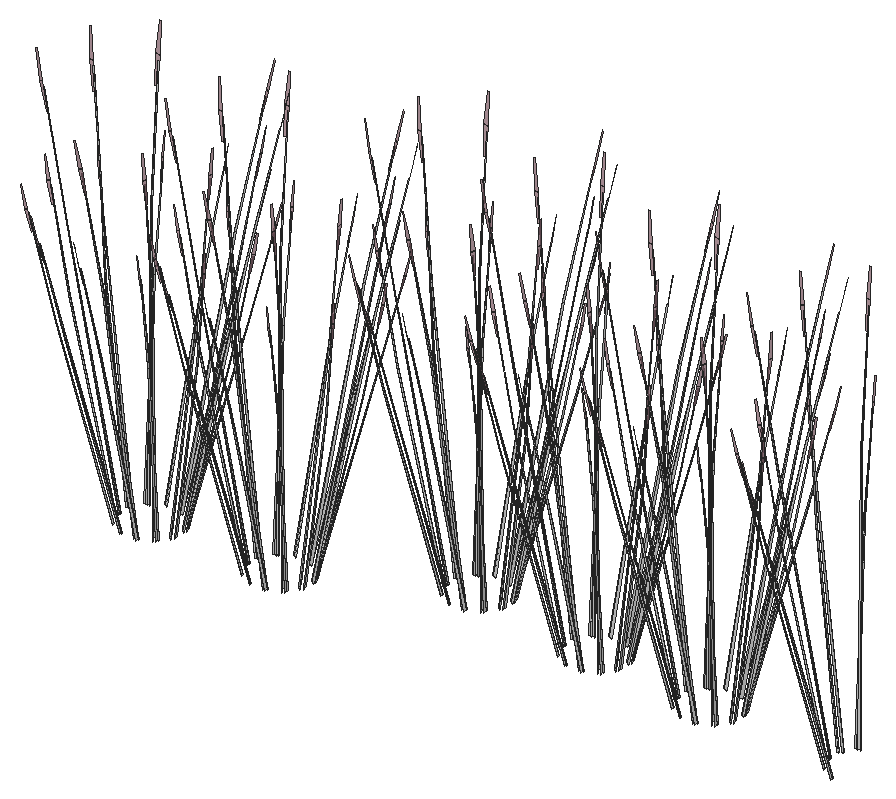
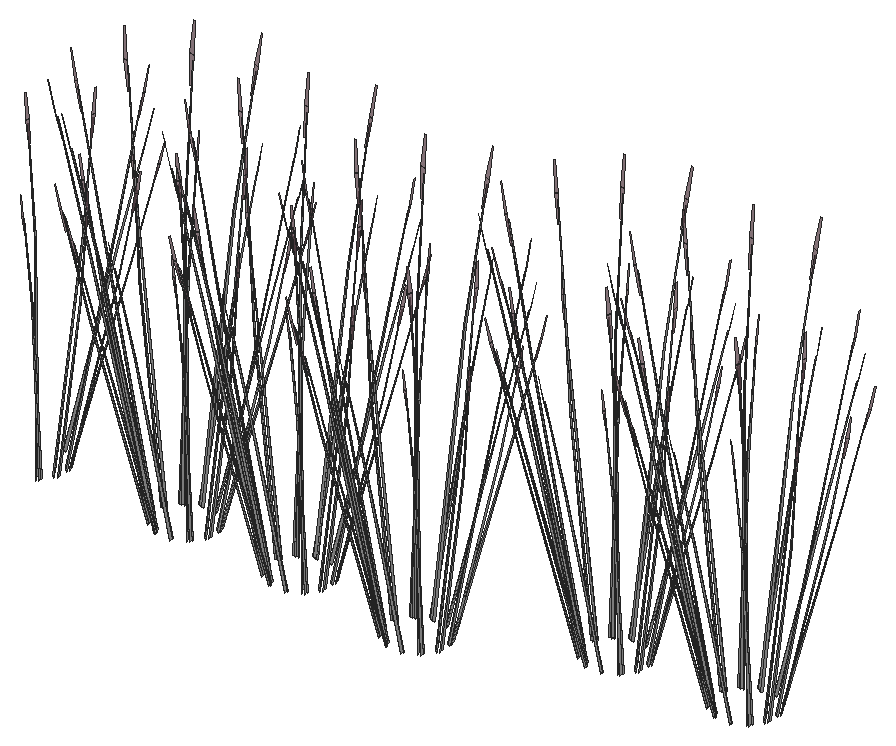
# SketchUp Ruby script. Lengths in inches.
U = 1.inch
M = Sketchup.active_model
def pt(a) = Geom::Point3d.new(a.map { |v| v * U })
def face(e, loops, mat)
  f = e.add_face(loops[0].map { |a| pt(a) })
  loops[1..].each { |l| e.add_face(l.map { |a| pt(a) }).erase! }
  f.material = f.back_material = mat if mat
  f
end
# faces: each face lists its corners as indices into pts; further lists are holes
def faces(e, pts, list, mat = nil) = list.each { |f| face(e, (f[0].is_a?(Array) ? f : [f]).map { |l| l.map { |i| pts[i] } }, mat) }
# xy, xz, yz: faces in a plane at the given z, y or x. An outline is a flat list of corners, or four numbers for a rectangle; further outlines are holes
def ring(l) = l.size == 4 ? [[l[0], l[1]], [l[2], l[1]], [l[2], l[3]], [l[0], l[3]]] : l.each_slice(2).to_a
def flat(e, list, mat, &to3) = list.each { |f| face(e, (f[0].is_a?(Array) ? f : [f]).map { |l| ring(l).map { |u, v| to3.(u, v) } }, mat) }
def xy(e, z, list, mat = nil) = flat(e, list, mat) { |x, y| [x, y, z] }
def xz(e, y, list, mat = nil) = flat(e, list, mat) { |x, z| [x, y, z] }
def yz(e, x, list, mat = nil) = flat(e, list, mat) { |y, z| [x, y, z] }
def lines(e, pts, list) = list.each { |a, b| e.add_line(pt(pts[a]), pt(pts[b])) }
# prism: a flat outline (further loops are holes) pulled along v
def prism(e, loops, v, mat = nil)
  f = face(e, loops, mat); d = Geom::Vector3d.new(v.map { |x| x * U })
  f.pushpull(f.normal.samedirection?(d) ? d.length : -d.length)
end
def box(e, o, s, mat = nil) = prism(e, [[o, [o[0] + s[0], o[1], o[2]], [o[0] + s[0], o[1] + s[1], o[2]], [o[0], o[1] + s[1], o[2]]]], [0, 0, s[2]], mat)
def at(x, y, z, deg = 0) = Geom::Transformation.translation(pt([x, y, z])) * Geom::Transformation.rotation(ORIGIN, Z_AXIS, deg.degrees)
def axes(o, x, y, z) = Geom::Transformation.new([*x, 0, *y, 0, *z, 0, *pt(o).to_a, 1])
def part(name) = M.definitions.add(name)
# library, detail: a bought-in or finely detailed component or shape, given as its bounding box
def library(name, o, s) = part(name).tap { |d| box(d.entities, o, s) }
def detail(e, o, s) = box(e.add_group.entities, o, s)
def put(e, d, t, mat = nil) = e.add_instance(d, t).tap { |i| i.material = mat if mat }
def group(e, t, mat = nil) = e.add_group.tap { |g| g.transformation = t; g.material = mat if mat }.entities
root = M.entities
M.materials.add("LightPink_Translucent").color = [144, 107, 117]
M.materials["LightPink_Translucent"].alpha = 0.75
M.materials.add("[_0053_Ivory_]").color = [200, 200, 200]
c1 = part("blade")
p = [[2.15,0.21,22],[0,0.17,0],[0.09,0.45,0],[2.18,0.31,22],[2.29,0.31,22],[0.38,0.45,0],
  [2.48,0.24,33],[2.49,0.24,33],[2.48,0.22,33]]
faces(c1.entities,p,[[0,1,2,3],[4,5,2,3],[6,3,4,7],[8,0,3,6]])
c2 = part("seeds")
p = [[0.3,-0.1,1.38],[-0.01,-0.03,1.59],[-0.01,-0.03,0.03],[0.14,-0.07,-0.07],[0.29,-0.03,3],[0.15,0.01,3.11]]
faces(c2.entities,p,[[0,1,2,3],[1,0,4,5]],"LightPink_Translucent")
c3 = part("blade with seeds")
put(c3.entities,c1,at(0,0,0))
put(c3.entities,c2,axes([2.4,0.25,30.99],[1.5799,-0.05474,1.17369],[-0.12525,1.92788,0.29478],[-0.07173,-0.02425,1.56792]))
put(root,c3,axes([417.64,97.95,131.39],[0.17159,-0.57338,0.48003],[0.56413,0.19607,0.3958],[-0.22185,0.03446,0.9933]),"[_0053_Ivory_]")
put(root,c3,axes([417.59,97.8,131.38],[-0.22307,-0.42878,0.0643],[0.40677,-0.20987,0.50621],[-0.17931,0.04141,0.77189]),"[_0053_Ivory_]")
put(root,c3,axes([417.77,99.38,131.39],[-0.15063,-0.57876,0.48003],[0.59087,-0.10045,0.3958],[-0.17414,0.13612,0.9933]),"[_0053_Ivory_]")
put(root,c3,axes([417.66,99.27,131.38],[-0.41695,-0.26447,0.0643],[0.24275,-0.37662,0.50621],[-0.13368,0.12176,0.77189]),"[_0053_Ivory_]")
put(root,c3,axes([418.31,96.5,131.38],[0.03058,-0.47819,0.0643],[0.4618,0.01311,0.50621],[-0.1769,-0.05004,0.77189]),"[_0053_Ivory_]")
put(root,c3,axes([418.64,100.55,131.39],[-0.43249,-0.42907,0.48003],[0.45929,-0.37004,0.3958],[-0.07978,0.2013,0.9933]),"[_0053_Ivory_]")
put(root,c3,axes([418.48,100.51,131.38],[-0.49911,-0.0293,0.0643],[0.01368,-0.44245,0.50621],[-0.05223,0.16948,0.77189]),"[_0053_Ivory_]")
put(root,c3,axes([419.6,95.71,131.38],[0.27604,-0.39948,0.0643],[0.39309,0.23258,0.50621],[-0.12709,-0.12808,0.77189]),"[_0053_Ivory_]")
put(root,c3,axes([419.84,101.2,131.38],[-0.44753,0.21372,0.0643],[-0.21905,-0.38973,0.50621],[0.04322,0.1718,0.77189]),"[_0053_Ivory_]")
put(root,c3,axes([421.14,95.65,131.38],[0.44753,-0.21372,0.0643],[0.21905,0.38973,0.50621],[-0.04322,-0.1718,0.77189]),"[_0053_Ivory_]")
put(root,c3,axes([420.98,95.7,131.39],[0.59846,0.1644,0.48003],[-0.20464,0.54049,0.3958],[-0.03596,-0.21255,0.9933]),"[_0053_Ivory_]")
put(root,c3,axes([421.48,101.02,131.39],[-0.60408,0.14432,0.48003],[-0.10484,-0.56611,0.3958],[0.14207,0.16684,0.9933]),"[_0053_Ivory_]")
put(root,c3,axes([421.37,101.14,131.38],[-0.27604,0.39948,0.0643],[-0.39309,-0.23258,0.50621],[0.12709,0.12808,0.77189]),"[_0053_Ivory_]")
put(root,c3,axes([422.49,96.34,131.38],[0.49911,0.0293,0.0643],[-0.01368,0.44245,0.50621],[0.05223,-0.16948,0.77189]),"[_0053_Ivory_]")
put(root,c3,axes([422.34,96.3,131.39],[0.43249,0.42907,0.48003],[-0.45929,0.37004,0.3958],[0.07978,-0.2013,0.9933]),"[_0053_Ivory_]")
put(root,c3,axes([422.67,100.35,131.38],[-0.03058,0.47819,0.0643],[-0.4618,-0.01311,0.50621],[0.1769,0.05004,0.77189]),"[_0053_Ivory_]")
put(root,c3,axes([422.71,100.2,131.39],[-0.44783,0.41436,0.48003],[-0.38623,-0.44004,0.3958],[0.21011,0.07643,0.9933]),"[_0053_Ivory_]")
put(root,c3,axes([429.85,97.95,131.39],[0.17159,-0.57338,0.48003],[0.56413,0.19607,0.3958],[-0.22185,0.03446,0.9933]),"[_0053_Ivory_]")
put(root,c3,axes([423.32,97.58,131.38],[0.41695,0.26447,0.0643],[-0.24275,0.37662,0.50621],[0.13368,-0.12176,0.77189]),"[_0053_Ivory_]")
put(root,c3,axes([429.81,97.8,131.38],[-0.22307,-0.42878,0.0643],[0.40677,-0.20987,0.50621],[-0.17931,0.04141,0.77189]),"[_0053_Ivory_]")
put(root,c3,axes([423.2,97.47,131.39],[0.15063,0.57876,0.48003],[-0.59087,0.10045,0.3958],[0.17414,-0.13612,0.9933]),"[_0053_Ivory_]")
put(root,c3,axes([429.99,99.38,131.39],[-0.15063,-0.57876,0.48003],[0.59087,-0.10045,0.3958],[-0.17414,0.13612,0.9933]),"[_0053_Ivory_]")
put(root,c3,axes([423.38,99.05,131.38],[0.22307,0.42878,0.0643],[-0.40677,0.20987,0.50621],[0.17931,-0.04141,0.77189]),"[_0053_Ivory_]")
put(root,c3,axes([429.87,99.27,131.38],[-0.41695,-0.26447,0.0643],[0.24275,-0.37662,0.50621],[-0.13368,0.12176,0.77189]),"[_0053_Ivory_]")
put(root,c3,axes([423.33,98.9,131.39],[-0.17159,0.57338,0.48003],[-0.56413,-0.19607,0.3958],[0.22185,-0.03446,0.9933]),"[_0053_Ivory_]")
put(root,c3,axes([430.52,96.5,131.38],[0.03058,-0.47819,0.0643],[0.4618,0.01311,0.50621],[-0.1769,-0.05004,0.77189]),"[_0053_Ivory_]")
put(root,c3,axes([430.85,100.55,131.39],[-0.43249,-0.42907,0.48003],[0.45929,-0.37004,0.3958],[-0.07978,0.2013,0.9933]),"[_0053_Ivory_]")
put(root,c3,axes([430.69,100.51,131.38],[-0.49911,-0.0293,0.0643],[0.01368,-0.44245,0.50621],[-0.05223,0.16948,0.77189]),"[_0053_Ivory_]")
put(root,c3,axes([431.82,95.71,131.38],[0.27604,-0.39948,0.0643],[0.39309,0.23258,0.50621],[-0.12709,-0.12808,0.77189]),"[_0053_Ivory_]")
put(root,c3,axes([432.05,101.2,131.38],[-0.44753,0.21372,0.0643],[-0.21905,-0.38973,0.50621],[0.04322,0.1718,0.77189]),"[_0053_Ivory_]")
put(root,c3,axes([433.35,95.65,131.38],[0.44753,-0.21372,0.0643],[0.21905,0.38973,0.50621],[-0.04322,-0.1718,0.77189]),"[_0053_Ivory_]")
put(root,c3,axes([433.19,95.7,131.39],[0.59846,0.1644,0.48003],[-0.20464,0.54049,0.3958],[-0.03596,-0.21255,0.9933]),"[_0053_Ivory_]")
put(root,c3,axes([433.7,101.02,131.39],[-0.60408,0.14432,0.48003],[-0.10484,-0.56611,0.3958],[0.14207,0.16684,0.9933]),"[_0053_Ivory_]")
put(root,c3,axes([433.58,101.14,131.38],[-0.27604,0.39948,0.0643],[-0.39309,-0.23258,0.50621],[0.12709,0.12808,0.77189]),"[_0053_Ivory_]")
put(root,c3,axes([434.71,96.34,131.38],[0.49911,0.0293,0.0643],[-0.01368,0.44245,0.50621],[0.05223,-0.16948,0.77189]),"[_0053_Ivory_]")
put(root,c3,axes([434.55,96.3,131.39],[0.43249,0.42907,0.48003],[-0.45929,0.37004,0.3958],[0.07978,-0.2013,0.9933]),"[_0053_Ivory_]")
put(root,c3,axes([434.88,100.35,131.38],[-0.03058,0.47819,0.0643],[-0.4618,-0.01311,0.50621],[0.1769,0.05004,0.77189]),"[_0053_Ivory_]")
put(root,c3,axes([434.92,100.2,131.39],[-0.44783,0.41436,0.48003],[-0.38623,-0.44004,0.3958],[0.21011,0.07643,0.9933]),"[_0053_Ivory_]")
put(root,c3,axes([435.53,97.58,131.38],[0.41695,0.26447,0.0643],[-0.24275,0.37662,0.50621],[0.13368,-0.12176,0.77189]),"[_0053_Ivory_]")
put(root,c3,axes([435.41,97.47,131.39],[0.15063,0.57876,0.48003],[-0.59087,0.10045,0.3958],[0.17414,-0.13612,0.9933]),"[_0053_Ivory_]")
put(root,c3,axes([435.59,99.05,131.38],[0.22307,0.42878,0.0643],[-0.40677,0.20987,0.50621],[0.17931,-0.04141,0.77189]),"[_0053_Ivory_]")
put(root,c3,axes([435.55,98.9,131.39],[-0.17159,0.57338,0.48003],[-0.56413,-0.19607,0.3958],[0.22185,-0.03446,0.9933]),"[_0053_Ivory_]")
put(root,c3,axes([443.25,104.76,131.39],[0.17159,-0.57338,0.48003],[0.56413,0.19607,0.3958],[-0.22185,0.03446,0.9933]),"[_0053_Ivory_]")
put(root,c3,axes([443.21,104.61,131.38],[-0.22307,-0.42878,0.0643],[0.40677,-0.20987,0.50621],[-0.17931,0.04141,0.77189]),"[_0053_Ivory_]")
put(root,c3,axes([443.39,106.19,131.39],[-0.15063,-0.57876,0.48003],[0.59087,-0.10045,0.3958],[-0.17414,0.13612,0.9933]),"[_0053_Ivory_]")
put(root,c3,axes([443.27,106.08,131.38],[-0.41695,-0.26447,0.0643],[0.24275,-0.37662,0.50621],[-0.13368,0.12176,0.77189]),"[_0053_Ivory_]")
put(root,c3,axes([443.92,103.31,131.38],[0.03058,-0.47819,0.0643],[0.4618,0.01311,0.50621],[-0.1769,-0.05004,0.77189]),"[_0053_Ivory_]")
put(root,c3,axes([444.25,107.36,131.39],[-0.43249,-0.42907,0.48003],[0.45929,-0.37004,0.3958],[-0.07978,0.2013,0.9933]),"[_0053_Ivory_]")
put(root,c3,axes([444.09,107.32,131.38],[-0.49911,-0.0293,0.0643],[0.01368,-0.44245,0.50621],[-0.05223,0.16948,0.77189]),"[_0053_Ivory_]")
put(root,c3,axes([445.22,102.52,131.38],[0.27604,-0.39948,0.0643],[0.39309,0.23258,0.50621],[-0.12709,-0.12808,0.77189]),"[_0053_Ivory_]")
put(root,c3,axes([445.45,108.01,131.38],[-0.44753,0.21372,0.0643],[-0.21905,-0.38973,0.50621],[0.04322,0.1718,0.77189]),"[_0053_Ivory_]")
put(root,c3,axes([446.75,102.46,131.38],[0.44753,-0.21372,0.0643],[0.21905,0.38973,0.50621],[-0.04322,-0.1718,0.77189]),"[_0053_Ivory_]")
put(root,c3,axes([446.59,102.5,131.39],[0.59846,0.1644,0.48003],[-0.20464,0.54049,0.3958],[-0.03596,-0.21255,0.9933]),"[_0053_Ivory_]")
put(root,c3,axes([447.1,107.83,131.39],[-0.60408,0.14432,0.48003],[-0.10484,-0.56611,0.3958],[0.14207,0.16684,0.9933]),"[_0053_Ivory_]")
put(root,c3,axes([446.99,107.95,131.38],[-0.27604,0.39948,0.0643],[-0.39309,-0.23258,0.50621],[0.12709,0.12808,0.77189]),"[_0053_Ivory_]")
put(root,c3,axes([448.11,103.15,131.38],[0.49911,0.0293,0.0643],[-0.01368,0.44245,0.50621],[0.05223,-0.16948,0.77189]),"[_0053_Ivory_]")
put(root,c3,axes([447.95,103.11,131.39],[0.43249,0.42907,0.48003],[-0.45929,0.37004,0.3958],[0.07978,-0.2013,0.9933]),"[_0053_Ivory_]")
put(root,c3,axes([448.28,107.16,131.38],[-0.03058,0.47819,0.0643],[-0.4618,-0.01311,0.50621],[0.1769,0.05004,0.77189]),"[_0053_Ivory_]")
put(root,c3,axes([448.32,107.01,131.39],[-0.44783,0.41436,0.48003],[-0.38623,-0.44004,0.3958],[0.21011,0.07643,0.9933]),"[_0053_Ivory_]")
put(root,c3,axes([448.93,104.39,131.38],[0.41695,0.26447,0.0643],[-0.24275,0.37662,0.50621],[0.13368,-0.12176,0.77189]),"[_0053_Ivory_]")
put(root,c3,axes([448.82,104.28,131.39],[0.15063,0.57876,0.48003],[-0.59087,0.10045,0.3958],[0.17414,-0.13612,0.9933]),"[_0053_Ivory_]")
put(root,c3,axes([455.74,102.94,131.39],[0.17159,-0.57338,0.48003],[0.56413,0.19607,0.3958],[-0.22185,0.03446,0.9933]),"[_0053_Ivory_]")
put(root,c3,axes([455.69,102.79,131.38],[-0.22307,-0.42878,0.0643],[0.40677,-0.20987,0.50621],[-0.17931,0.04141,0.77189]),"[_0053_Ivory_]")
put(root,c3,axes([448.99,105.86,131.38],[0.22307,0.42878,0.0643],[-0.40677,0.20987,0.50621],[0.17931,-0.04141,0.77189]),"[_0053_Ivory_]")
put(root,c3,axes([448.95,105.71,131.39],[-0.17159,0.57338,0.48003],[-0.56413,-0.19607,0.3958],[0.22185,-0.03446,0.9933]),"[_0053_Ivory_]")
put(root,c3,axes([455.87,104.37,131.39],[-0.15063,-0.57876,0.48003],[0.59087,-0.10045,0.3958],[-0.17414,0.13612,0.9933]),"[_0053_Ivory_]")
put(root,c3,axes([455.75,104.26,131.38],[-0.41695,-0.26447,0.0643],[0.24275,-0.37662,0.50621],[-0.13368,0.12176,0.77189]),"[_0053_Ivory_]")
put(root,c3,axes([456.4,101.49,131.38],[0.03058,-0.47819,0.0643],[0.4618,0.01311,0.50621],[-0.1769,-0.05004,0.77189]),"[_0053_Ivory_]")
put(root,c3,axes([456.73,105.54,131.39],[-0.43249,-0.42907,0.48003],[0.45929,-0.37004,0.3958],[-0.07978,0.2013,0.9933]),"[_0053_Ivory_]")
put(root,c3,axes([456.58,105.5,131.38],[-0.49911,-0.0293,0.0643],[0.01368,-0.44245,0.50621],[-0.05223,0.16948,0.77189]),"[_0053_Ivory_]")
put(root,c3,axes([457.7,100.7,131.38],[0.27604,-0.39948,0.0643],[0.39309,0.23258,0.50621],[-0.12709,-0.12808,0.77189]),"[_0053_Ivory_]")
put(root,c3,axes([457.93,106.1875,131.38],[-0.44753,0.21372,0.0643],[-0.21905,-0.38973,0.50621],[0.04322,0.1718,0.77189]),"[_0053_Ivory_]")
put(root,c3,axes([459.23,100.64,131.38],[0.44753,-0.21372,0.0643],[0.21905,0.38973,0.50621],[-0.04322,-0.1718,0.77189]),"[_0053_Ivory_]")
put(root,c3,axes([459.08,100.6875,131.39],[0.59846,0.1644,0.48003],[-0.20464,0.54049,0.3958],[-0.03596,-0.21255,0.9933]),"[_0053_Ivory_]")
put(root,c3,axes([459.58,106.02,131.39],[-0.60408,0.14432,0.48003],[-0.10484,-0.56611,0.3958],[0.14207,0.16684,0.9933]),"[_0053_Ivory_]")
put(root,c3,axes([459.47,106.13,131.38],[-0.27604,0.39948,0.0643],[-0.39309,-0.23258,0.50621],[0.12709,0.12808,0.77189]),"[_0053_Ivory_]")
put(root,c3,axes([460.59,101.33,131.38],[0.49911,0.0293,0.0643],[-0.01368,0.44245,0.50621],[0.05223,-0.16948,0.77189]),"[_0053_Ivory_]")
put(root,c3,axes([460.43,101.29,131.39],[0.43249,0.42907,0.48003],[-0.45929,0.37004,0.3958],[0.07978,-0.2013,0.9933]),"[_0053_Ivory_]")
put(root,c3,axes([467.25,102.09,131.39],[0.17159,-0.57338,0.48003],[0.56413,0.19607,0.3958],[-0.22185,0.03446,0.9933]),"[_0053_Ivory_]")
put(root,c3,axes([467.21,101.94,131.38],[-0.22307,-0.42878,0.0643],[0.40677,-0.20987,0.50621],[-0.17931,0.04141,0.77189]),"[_0053_Ivory_]")
put(root,c3,axes([460.76,105.34,131.38],[-0.03058,0.47819,0.0643],[-0.4618,-0.01311,0.50621],[0.1769,0.05004,0.77189]),"[_0053_Ivory_]")
put(root,c3,axes([460.81,105.1875,131.39],[-0.44783,0.41436,0.48003],[-0.38623,-0.44004,0.3958],[0.21011,0.07643,0.9933]),"[_0053_Ivory_]")
put(root,c3,axes([467.38,103.52,131.39],[-0.15063,-0.57876,0.48003],[0.59087,-0.10045,0.3958],[-0.17414,0.13612,0.9933]),"[_0053_Ivory_]")
put(root,c3,axes([467.27,103.4,131.38],[-0.41695,-0.26447,0.0643],[0.24275,-0.37662,0.50621],[-0.13368,0.12176,0.77189]),"[_0053_Ivory_]")
put(root,c3,axes([461.41,102.57,131.38],[0.41695,0.26447,0.0643],[-0.24275,0.37662,0.50621],[0.13368,-0.12176,0.77189]),"[_0053_Ivory_]")
put(root,c3,axes([461.3,102.46,131.39],[0.15063,0.57876,0.48003],[-0.59087,0.10045,0.3958],[0.17414,-0.13612,0.9933]),"[_0053_Ivory_]")
put(root,c3,axes([467.92,100.63,131.38],[0.03058,-0.47819,0.0643],[0.4618,0.01311,0.50621],[-0.1769,-0.05004,0.77189]),"[_0053_Ivory_]")
put(root,c3,axes([461.48,104.04,131.38],[0.22307,0.42878,0.0643],[-0.40677,0.20987,0.50621],[0.17931,-0.04141,0.77189]),"[_0053_Ivory_]")
put(root,c3,axes([461.43,103.89,131.39],[-0.17159,0.57338,0.48003],[-0.56413,-0.19607,0.3958],[0.22185,-0.03446,0.9933]),"[_0053_Ivory_]")
put(root,c3,axes([468.25,104.6875,131.39],[-0.43249,-0.42907,0.48003],[0.45929,-0.37004,0.3958],[-0.07978,0.2013,0.9933]),"[_0053_Ivory_]")
put(root,c3,axes([468.09,104.65,131.38],[-0.49911,-0.0293,0.0643],[0.01368,-0.44245,0.50621],[-0.05223,0.16948,0.77189]),"[_0053_Ivory_]")
put(root,c3,axes([469.22,99.85,131.38],[0.27604,-0.39948,0.0643],[0.39309,0.23258,0.50621],[-0.12709,-0.12808,0.77189]),"[_0053_Ivory_]")
put(root,c3,axes([469.45,105.33,131.38],[-0.44753,0.21372,0.0643],[-0.21905,-0.38973,0.50621],[0.04322,0.1718,0.77189]),"[_0053_Ivory_]")
put(root,c3,axes([470.75,99.79,131.38],[0.44753,-0.21372,0.0643],[0.21905,0.38973,0.50621],[-0.04322,-0.1718,0.77189]),"[_0053_Ivory_]")
put(root,c3,axes([470.59,99.83,131.39],[0.59846,0.1644,0.48003],[-0.20464,0.54049,0.3958],[-0.03596,-0.21255,0.9933]),"[_0053_Ivory_]")
put(root,c3,axes([471.1,105.16,131.39],[-0.60408,0.14432,0.48003],[-0.10484,-0.56611,0.3958],[0.14207,0.16684,0.9933]),"[_0053_Ivory_]")
put(root,c3,axes([470.98,105.27,131.38],[-0.27604,0.39948,0.0643],[-0.39309,-0.23258,0.50621],[0.12709,0.12808,0.77189]),"[_0053_Ivory_]")
put(root,c3,axes([472.11,100.47,131.38],[0.49911,0.0293,0.0643],[-0.01368,0.44245,0.50621],[0.05223,-0.16948,0.77189]),"[_0053_Ivory_]")
put(root,c3,axes([471.95,100.43,131.39],[0.43249,0.42907,0.48003],[-0.45929,0.37004,0.3958],[0.07978,-0.2013,0.9933]),"[_0053_Ivory_]")
put(root,c3,axes([472.28,104.48,131.38],[-0.03058,0.47819,0.0643],[-0.4618,-0.01311,0.50621],[0.1769,0.05004,0.77189]),"[_0053_Ivory_]")
put(root,c3,axes([472.32,104.33,131.39],[-0.44783,0.41436,0.48003],[-0.38623,-0.44004,0.3958],[0.21011,0.07643,0.9933]),"[_0053_Ivory_]")
put(root,c3,axes([472.93,101.71,131.38],[0.41695,0.26447,0.0643],[-0.24275,0.37662,0.50621],[0.13368,-0.12176,0.77189]),"[_0053_Ivory_]")
put(root,c3,axes([472.8125,101.6,131.39],[0.15063,0.57876,0.48003],[-0.59087,0.10045,0.3958],[0.17414,-0.13612,0.9933]),"[_0053_Ivory_]")
put(root,c3,axes([472.99,103.18,131.38],[0.22307,0.42878,0.0643],[-0.40677,0.20987,0.50621],[0.17931,-0.04141,0.77189]),"[_0053_Ivory_]")
put(root,c3,axes([472.95,103.03,131.39],[-0.17159,0.57338,0.48003],[-0.56413,-0.19607,0.3958],[0.22185,-0.03446,0.9933]),"[_0053_Ivory_]")
put(root,c3,axes([481.74,101.88,131.39],[0.17159,-0.57338,0.48003],[0.56413,0.19607,0.3958],[-0.22185,0.03446,0.9933]),"[_0053_Ivory_]")
put(root,c3,axes([481.7,101.73,131.38],[-0.22307,-0.42878,0.0643],[0.40677,-0.20987,0.50621],[-0.17931,0.04141,0.77189]),"[_0053_Ivory_]")
put(root,c3,axes([481.875,103.31,131.39],[-0.15063,-0.57876,0.48003],[0.59087,-0.10045,0.3958],[-0.17414,0.13612,0.9933]),"[_0053_Ivory_]")
put(root,c3,axes([481.76,103.19,131.38],[-0.41695,-0.26447,0.0643],[0.24275,-0.37662,0.50621],[-0.13368,0.12176,0.77189]),"[_0053_Ivory_]")
put(root,c3,axes([482.41,100.42,131.38],[0.03058,-0.47819,0.0643],[0.4618,0.01311,0.50621],[-0.1769,-0.05004,0.77189]),"[_0053_Ivory_]")
put(root,c3,axes([482.74,104.48,131.39],[-0.43249,-0.42907,0.48003],[0.45929,-0.37004,0.3958],[-0.07978,0.2013,0.9933]),"[_0053_Ivory_]")
put(root,c3,axes([482.58,104.4375,131.38],[-0.49911,-0.0293,0.0643],[0.01368,-0.44245,0.50621],[-0.05223,0.16948,0.77189]),"[_0053_Ivory_]")
put(root,c3,axes([483.71,99.64,131.38],[0.27604,-0.39948,0.0643],[0.39309,0.23258,0.50621],[-0.12709,-0.12808,0.77189]),"[_0053_Ivory_]")
